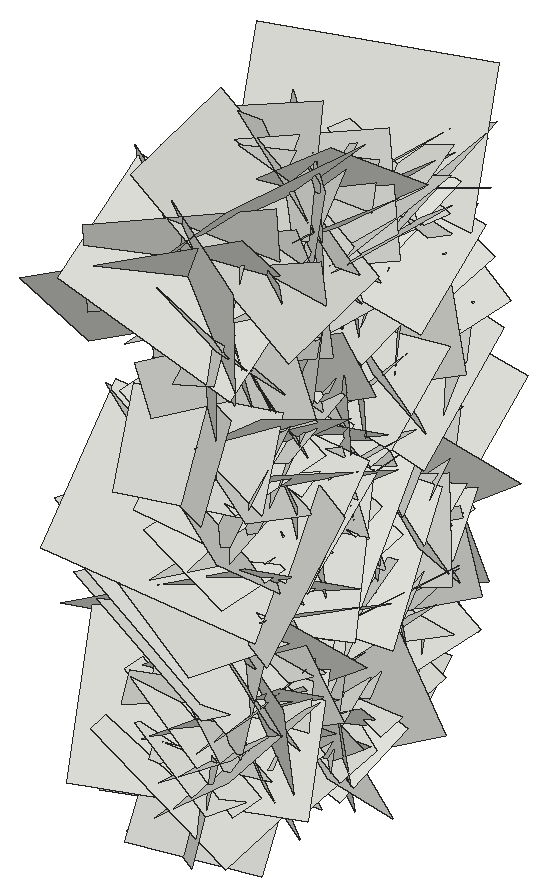
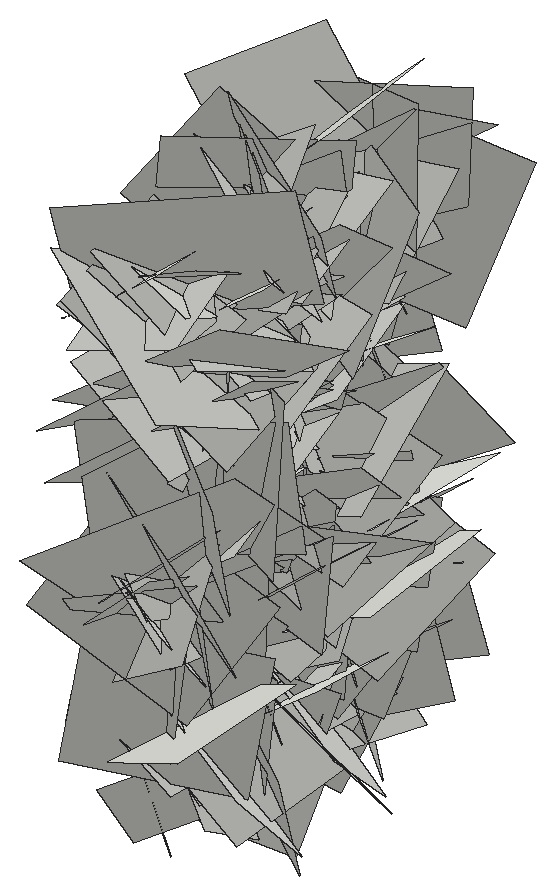
# SketchUp Ruby script. Lengths in inches.
U = 1.inch
M = Sketchup.active_model
def pt(a) = Geom::Point3d.new(a.map { |v| v * U })
def face(e, loops, mat)
  f = e.add_face(loops[0].map { |a| pt(a) })
  loops[1..].each { |l| e.add_face(l.map { |a| pt(a) }).erase! }
  f.material = f.back_material = mat if mat
  f
end
# faces: each face lists its corners as indices into pts; further lists are holes
def faces(e, pts, list, mat = nil) = list.each { |f| face(e, (f[0].is_a?(Array) ? f : [f]).map { |l| l.map { |i| pts[i] } }, mat) }
# xy, xz, yz: faces in a plane at the given z, y or x. An outline is a flat list of corners, or four numbers for a rectangle; further outlines are holes
def ring(l) = l.size == 4 ? [[l[0], l[1]], [l[2], l[1]], [l[2], l[3]], [l[0], l[3]]] : l.each_slice(2).to_a
def flat(e, list, mat, &to3) = list.each { |f| face(e, (f[0].is_a?(Array) ? f : [f]).map { |l| ring(l).map { |u, v| to3.(u, v) } }, mat) }
def xy(e, z, list, mat = nil) = flat(e, list, mat) { |x, y| [x, y, z] }
def xz(e, y, list, mat = nil) = flat(e, list, mat) { |x, z| [x, y, z] }
def yz(e, x, list, mat = nil) = flat(e, list, mat) { |y, z| [x, y, z] }
def lines(e, pts, list) = list.each { |a, b| e.add_line(pt(pts[a]), pt(pts[b])) }
# prism: a flat outline (further loops are holes) pulled along v
def prism(e, loops, v, mat = nil)
  f = face(e, loops, mat); d = Geom::Vector3d.new(v.map { |x| x * U })
  f.pushpull(f.normal.samedirection?(d) ? d.length : -d.length)
end
def box(e, o, s, mat = nil) = prism(e, [[o, [o[0] + s[0], o[1], o[2]], [o[0] + s[0], o[1] + s[1], o[2]], [o[0], o[1] + s[1], o[2]]]], [0, 0, s[2]], mat)
def at(x, y, z, deg = 0) = Geom::Transformation.translation(pt([x, y, z])) * Geom::Transformation.rotation(ORIGIN, Z_AXIS, deg.degrees)
def axes(o, x, y, z) = Geom::Transformation.new([*x, 0, *y, 0, *z, 0, *pt(o).to_a, 1])
def part(name) = M.definitions.add(name)
# library, detail: a bought-in or finely detailed component or shape, given as its bounding box
def library(name, o, s) = part(name).tap { |d| box(d.entities, o, s) }
def detail(e, o, s) = box(e.add_group.entities, o, s)
def put(e, d, t, mat = nil) = e.add_instance(d, t).tap { |i| i.material = mat if mat }
def group(e, t, mat = nil) = e.add_group.tap { |g| g.transformation = t; g.material = mat if mat }.entities
root = M.entities
c1 = part("Component\#6")
p = [[0.01,0,0],[0,3.24,4.54],[4.32,3.24,4.54],[4.33,0,0]]
faces(c1.entities,p,[[0,1,2,3]])
put(root,c1,axes([404.88,182.27,16.13],[-0.23771,-0.47409,1.27281],[-0.00404,1.29026,0.47991],[-1.43973,0.07465,-0.2115]))
put(root,c1,axes([404.88,189.11,8.53],[-0.25892,-1.11224,-0.53402],[-0.14932,-0.51568,1.13849],[-1.29927,0.28091,-0.02442]))
put(root,c1,axes([404.88,193.85,16.74],[-0.30124,-1.14539,-0.57535],[0.00001,-0.58933,1.17321],[-1.35869,0.25394,0.12757]))
put(root,c1,axes([404.88,184.58,6.82],[-0.16596,-1.29847,0.14138],[-0.0614,0.14916,1.30572],[-1.38315,0.14917,-0.07492]))
put(root,c1,axes([404.88,183.54,2.14],[-0.03864,0.84179,0.92004],[-0.33491,0.88417,-0.82148],[-1.27872,-0.257,0.18735]))
put(root,c1,axes([404.88,180.76,23.09],[-0.06995,0.91309,-0.96842],[-0.10566,-0.97028,-0.90805],[-1.4069,0.02747,0.11634]))
put(root,c1,axes([404.88,187.39,3.1875],[-0.10139,0.89849,0.89189],[-0.1671,0.87902,-0.90243],[-1.33152,-0.17873,0.04534]))
put(root,c1,axes([404.88,189.55,17.94],[-0.16397,-1.09761,-0.83604],[0.11999,-0.84854,1.09307],[-1.45761,0.05363,0.18403]))
put(root,c1,axes([404.88,193.03,3.2],[-0.23388,-1.096,0.27231],[-0.13541,0.2999,1.10354],[-1.1894,0.18138,-0.17918]))
put(root,c1,axes([404.88,184.34,4.6],[-0.11485,-1.15497,0.26483],[-0.19184,0.27894,1.14248],[-1.2413,0.06375,-0.20107]))
put(root,c1,axes([404.88,186.39,13.5625],[-0.22643,-0.80881,0.81079],[-0.0736,0.83241,0.81208],[-1.21171,0.10058,-0.20084]))
put(root,c1,axes([404.88,188.34,12.62],[-0.20954,0.481,1.15591],[0.07101,1.17261,-0.47649],[-1.32521,-0.01322,-0.2083]))
put(root,c1,axes([404.88,184,8.18],[0.02134,-1.06466,0.81449],[-0.04088,0.81378,1.06469],[-1.42032,-0.03942,-0.01841]))
put(root,c1,axes([404.88,184.23,21.55],[-0.30098,0.54789,0.85036],[-0.10123,0.86476,-0.58905],[-1.06749,-0.23649,-0.1839]))
put(root,c1,axes([404.88,183.88,15.08],[0.0404,1.11797,-0.62329],[-0.16276,-0.61507,-1.11262],[-1.34698,0.10785,0.11575]))
put(root,c1,axes([404.88,195.54,11.625],[-0.04246,-1.00606,-0.92627],[0.11693,-0.92602,1.00103],[-1.44486,-0.04538,0.10823]))
put(root,c1,axes([404.88,186.02,17.55],[-0.12484,-0.91824,0.67786],[-0.09261,0.68671,0.91505],[-1.20627,0.04231,-0.14041]))
put(root,c1,axes([404.88,185.87,11.99],[-0.00632,-0.88407,-1.06115],[0.10628,-1.05864,0.88141],[-1.46017,-0.07323,0.06874]))
put(root,c1,axes([404.88,192.77,15.58],[-0.03721,-0.16955,-1.17702],[-0.1418,-1.1695,0.17246],[-1.25252,0.13744,0.01545]))
put(root,c1,axes([404.88,186.66,10.07],[0.09303,-0.2424,1.37134],[0.00293,1.37409,0.24271],[-1.47615,-0.01254,0.08691]))
put(root,c1,axes([404.88,182.38,2.76],[-0.16715,0.82367,0.72398],[-0.09449,0.71938,-0.83785],[-1.15857,-0.1775,-0.03612]))
put(root,c1,axes([404.88,185.25,0.97],[-0.15144,0.45294,1.0525],[-0.02813,1.05906,-0.45936],[-1.21425,-0.08102,-0.12063]))
put(root,c1,axes([404.88,184.5,10.44],[-0.20009,0.552,-0.98447],[0.02572,-0.99592,-0.56307],[-1.1961,-0.11375,0.15258]))
put(root,c1,axes([404.88,180.93,10.86],[0.17521,1.15715,-0.62152],[-0.20897,-0.59747,-1.1648],[-1.37654,0.23798,0.09772]))
put(root,c1,axes([404.88,185.31,6.45],[0.03902,-0.20515,1.15818],[-0.22164,1.13915,0.20842],[-1.22693,-0.21231,-0.00082]))
put(root,c1,axes([404.88,183.02,16.38],[0.02893,-0.8566,0.75588],[-0.26219,0.73373,0.84043],[-1.18223,-0.18368,-0.16789]))
put(root,c1,axes([404.88,190.12,11.53],[0.21117,-0.99907,-0.90649],[-0.1512,-0.92678,0.99009],[-1.42194,-0.04983,-0.2399]))
put(root,c1,axes([404.88,188.7,21.97],[-0.14471,1.28216,-0.28655],[0.25359,-0.25902,-1.27293],[-1.36933,-0.18346,-0.20546]))
put(root,c1,axes([404.88,189.36,1.43],[0.09807,-1.35815,-0.14277],[0.05055,-0.1398,1.36078],[-1.44669,-0.09695,0.03787]))
put(root,c1,axes([404.88,194.04,23.84],[0.15699,-0.54259,-1.24113],[-0.03696,-1.24964,0.54215],[-1.43535,-0.02717,-0.14971]))
put(root,c1,axes([404.88,188.23,7.57],[-0.0913,-1.12353,0.75234],[0.27462,0.72618,1.11413],[-1.40673,0.21468,0.16867]))
put(root,c1,axes([404.88,192.17,8.01],[-0.17438,0.53527,-0.89237],[-0.02164,-0.90494,-0.53904],[-1.10282,-0.06688,0.15168]))
put(root,c1,axes([404.88,182.53,23.48],[-0.24403,0.37129,-0.99391],[0.1038,-1.00526,-0.39821],[-1.11985,-0.17408,0.17968]))
put(root,c1,axes([404.88,182.44,13.63],[0.1579,1.28482,-0.45217],[0.02165,-0.45692,-1.2916],[-1.44363,0.13368,-0.06883]))
put(root,c1,axes([404.88,189.08,9.2],[0.13088,0.55221,1.09741],[-0.12619,1.10312,-0.54169],[-1.29609,-0.05164,0.16356]))
put(root,c1,axes([404.88,187.9375,5.11],[-0.04973,-1.23753,-0.07043],[0.13139,-0.07481,1.23194],[-1.30732,0.03956,0.12649]))
put(root,c1,axes([400.91,190.35,18.26],[-0.16101,-0.65287,0.16772],[-0.08445,0.18811,0.66008],[0.7095,-0.12576,0.11663]))
put(root,c1,axes([404.88,186.43,6.6],[0.00451,1.27416,-0.10814],[0.14001,-0.108,-1.26731],[-1.34821,-0.00695,-0.13197]))
put(root,c1,axes([404.88,185.36,5.79],[-0.02078,-1.22604,-0.15411],[0.11589,-0.15525,1.22117],[-1.3047,0.00574,0.11093]))
put(root,c1,axes([404.88,188.68,19.83],[0.08458,1.11358,0.50301],[0.01593,0.50315,-1.11627],[-1.29513,0.07891,0.01912]))
put(root,c1,axes([404.88,186.13,19.34],[-0.13168,0.96657,0.23982],[-0.01085,0.24043,-0.97432],[-1.05558,-0.12304,-0.0199]))
put(root,c1,axes([400.91,191.11,1.26],[-0.04561,-0.57908,-0.31344],[-0.1156,-0.3035,0.57569],[0.68833,-0.08935,0.07592]))
put(root,c1,axes([404.88,187.26,9.21],[-0.06299,-0.71122,-0.64775],[-0.16214,-0.63375,0.70987],[-1.00673,0.14657,-0.0738]))
put(root,c1,axes([404.88,187.48,17.59],[0.04794,-0.78864,0.66349],[-0.19289,0.64758,0.78214],[-1.07529,-0.15133,-0.11072]))
put(root,c1,axes([404.88,180.4,17.125],[0.23878,-0.31981,1.17522],[-0.15258,1.17979,0.34864],[-1.28199,-0.19998,0.17739]))
put(root,c1,axes([404.88,185.11,13.22],[-0.08906,-0.95701,-0.12674],[-0.0585,-0.12225,0.95969],[-1.02162,0.09043,-0.0439]))
put(root,c1,axes([404.88,191.125,9.45],[0.23474,-0.88576,-0.93612],[-0.00151,-0.95001,0.89856],[-1.36608,-0.15116,-0.16185]))
put(root,c1,axes([404.88,184.05,20.67],[-0.10102,0.73684,0.6989],[0.04073,0.70408,-0.73707],[-1.07574,-0.04254,-0.09354]))
put(root,c1,axes([404.88,181.08,20.02],[0.00536,1.00575,0.03656],[-0.10796,0.03689,-1.00058],[-1.06133,0.00133,0.10197]))
put(root,c1,axes([404.88,185.52,6.2],[0.2751,-0.65276,-1.16933],[0.03559,-1.18754,0.67037],[-1.41909,-0.15632,-0.20987]))
put(root,c1,axes([400.91,188.8,6.44],[-0.14743,-0.18272,-0.74199],[-0.06403,-0.74919,0.19581],[0.80747,-0.09277,-0.11994]))
put(root,c1,axes([404.88,179.32,18.3],[-0.15069,0.54422,0.74866],[0.00735,0.75804,-0.54972],[-0.98107,-0.07791,-0.11911]))
put(root,c1,axes([404.88,184.31,4.6],[-0.1576,-0.1516,-1.0147],[0.15202,-1.0183,0.13112],[-1.07684,-0.12157,0.16702]))
put(root,c1,axes([400.91,186.3,8.38],[0.07617,0.47932,0.41871],[-0.13681,0.42359,-0.46276],[0.66062,0.03245,-0.14411]))
put(root,c1,axes([404.88,184.41,20.14],[0.03821,-1.03167,-0.60174],[0.15497,-0.59368,1.0266],[-1.25647,-0.1046,0.10832]))
put(root,c1,axes([404.88,194.3,13.93],[0.22437,-1.23478,-0.60854],[0.19245,-0.58527,1.25072],[-1.44644,-0.26941,0.07201]))
put(root,c1,axes([400.91,187.98,11.49],[-0.12716,0.81746,0.20835],[-0.15,0.18797,-0.81896],[0.88154,0.1499,-0.10929]))
put(root,c1,axes([400.91,186.0625,6.1],[-0.08854,0.52684,0.45627],[0.00383,0.45985,-0.53032],[0.73876,0.06076,0.05744]))
put(root,c1,axes([404.88,181.29,16.68],[-0.08133,-0.245,0.96212],[0.05676,0.96256,0.24939],[-1.05086,0.07095,-0.06099]))
put(root,c1,axes([404.88,184.19,13.53],[-0.08078,-0.49886,0.79857],[-0.01528,0.8017,0.49945],[-0.99796,0.02811,-0.07229]))
put(root,c1,axes([404.88,187.61,11.62],[0.28203,-0.58282,-1.12773],[-0.01249,-1.15332,0.59327],[-1.34554,-0.11146,-0.24188]))
put(root,c1,axes([400.91,183.1,18.89],[-0.1435,0.17311,-0.85276],[-0.14536,-0.85648,-0.1521],[0.91084,-0.10941,-0.15862]))
put(root,c1,axes([400.91,183.83,7.3125],[-0.02805,0.62389,-0.09529],[0.05665,-0.09282,-0.62253],[0.66659,0.03414,0.0489]))
put(root,c1,axes([404.88,184.51,1.15],[0.01173,-1.06899,-0.22188],[0.10644,-0.21996,1.06472],[-1.15237,-0.0312,0.09608]))
put(root,c1,axes([404.88,186.9375,3.03],[-0.11563,0.62873,-0.58509],[-0.05581,-0.59358,-0.62803],[-0.90867,-0.04354,0.11303]))
put(root,c1,axes([400.91,189.45,1.42],[0.1039,0.30381,0.53974],[-0.07033,0.54846,-0.29667],[0.65275,0.01074,-0.11787]))
put(root,c1,axes([400.91,184.54,3.47],[-0.05739,0.5962,-0.42459],[-0.0201,-0.42675,-0.59681],[0.77559,0.03305,-0.04688]))
put(root,c1,axes([404.88,185.64,19.96],[0.2349,1.07139,0.39402],[-0.08081,0.41437,-1.08385],[-1.20734,0.18072,0.1492]))
put(root,c1,axes([404.88,186.72,4.72],[0.08241,-0.91883,0.29273],[-0.13826,0.28096,0.91654],[-1.0128,-0.11312,-0.1013]))
put(root,c1,axes([404.88,190.33,17.67],[-0.17424,0.82504,0.17436],[0.04616,0.18571,-0.83769],[-0.89267,-0.15144,-0.07735]))
put(root,c1,axes([404.88,179.97,24.47],[0.23304,1.36821,0.06434],[0.25904,0.02493,-1.36533],[-1.42861,0.2277,-0.23708]))
put(root,c1,axes([400.91,184.43,15.42],[-0.12844,-0.04329,0.74472],[0.08874,0.74892,0.05716],[0.78574,-0.09166,0.11528]))
put(root,c1,axes([404.88,189.57,16.9],[-0.06471,0.53395,-0.71324],[-0.01751,-0.71546,-0.53421],[-0.94426,-0.02333,0.05878]))
put(root,c1,axes([404.88,191,16.96],[0.17643,-1.14926,-0.11809],[0.05518,-0.11173,1.16072],[-1.22339,-0.17078,0.03532]))
put(root,c1,axes([400.91,186.92,8.78],[-0.10246,-0.30095,0.75916],[-0.04625,0.76527,0.29782],[0.86439,0.00528,0.10592]))
put(root,c1,axes([404.88,180.14,11.99],[0.0212,0.75168,0.8023],[0.17372,0.79143,-0.74558],[-1.15236,0.13314,-0.09764]))
put(root,c1,axes([404.88,185.08,2.16],[-0.06404,-1.02262,-0.11109],[0.17979,-0.11966,1.00929],[-1.07543,0.04089,0.17535]))
put(root,c1,axes([404.88,187.17,12.95],[0.05814,-0.16279,1.09674],[0.14666,1.09051,0.15494],[-1.1661,0.12904,0.07417]))
put(root,c1,axes([404.88,187.85,22.99],[-0.09057,-0.06637,-0.91857],[0.07612,-0.92019,0.05981],[-0.97325,-0.06579,0.09016]))
put(root,c1,axes([400.91,183.375,2.21],[0.01982,-0.33114,-0.74136],[-0.16849,-0.7287,0.32148],[0.84401,-0.13769,0.08159]))
put(root,c1,axes([400.91,192.83,7.86],[0.1126,-0.65912,-0.17655],[-0.1088,-0.19208,0.65534],[0.71507,0.07456,0.12751]))
put(root,c1,axes([404.88,183.46,7.83],[0.1867,0.36795,-0.96583],[-0.13041,-0.96532,-0.39019],[-1.08777,0.17888,-0.11899]))
put(root,c1,axes([404.88,186.63,-0.64],[0.14781,-0.37723,1.01914],[0.01271,1.02797,0.37886],[-1.15185,-0.03706,0.13496]))
put(root,c1,axes([404.88,183.61,1.59],[-0.06331,-0.78644,0.46242],[0.03597,0.46118,0.7887],[-0.96639,0.06869,-0.00094]))
put(root,c1,axes([404.88,185.25,15.47],[-0.04372,0.77316,0.71524],[0.20224,0.70943,-0.75587],[-1.09798,0.09988,-0.16771]))
put(root,c1,axes([404.88,185.13,2.21],[-0.09174,0.69928,0.36],[-0.10121,0.35015,-0.7031],[-0.82753,-0.12035,0.04608]))
put(root,c1,axes([400.91,192.38,19.24],[0.04943,-0.7355,0.057],[-0.07325,0.05251,0.73407],[0.77853,0.05163,0.06545]))
put(root,c1,axes([404.88,181.6,11.88],[-0.05183,0.72565,0.67247],[0.15864,0.67097,-0.71314],[-1.03662,0.0664,-0.14276]))
put(root,c1,axes([400.91,185.26,12.26],[-0.159,0.84642,0.10737],[0.04855,0.11685,-0.85715],[0.9031,0.14274,0.06498]))
put(root,c1,axes([400.91,185.94,13.1875],[-0.12339,0.16979,-0.82402],[0.01755,-0.83125,-0.17361],[0.89164,0.03986,-0.11061]))
put(root,c1,axes([400.91,183.19,13.8],[-0.02762,0.65605,0.3231],[0.06014,0.32414,-0.6536],[0.77284,-0.00178,0.06241]))
put(root,c1,axes([404.88,184.53,11.29],[0.10396,-0.95246,0.37472],[0.04499,0.37989,0.95451],[-1.084,-0.07558,0.07555]))
put(root,c1,axes([404.88,192.08,20.31],[-0.05296,-0.67773,-0.30339],[-0.1724,-0.2867,0.66724],[-0.76797,0.11109,-0.12886]))
put(root,c1,axes([400.91,192.03,8.33],[-0.03388,0.22508,-0.86549],[-0.13142,-0.8588,-0.21876],[0.93879,-0.1121,-0.06186]))
put(root,c1,axes([400.91,185.14,8.49],[0.08576,-0.66072,-0.04627],[0.0456,-0.04128,0.66459],[0.70059,0.08356,-0.03759]))
put(root,c1,axes([400.91,183.28,17.73],[-0.09647,-0.26045,0.74001],[0.11879,0.73302,0.27177],[0.82305,-0.13632,0.04751]))
put(root,c1,axes([400.91,193.37,9.31],[-0.05697,-0.46717,-0.61186],[0.09106,-0.61316,0.46062],[0.81091,0.03603,-0.09471]))
put(root,c1,axes([400.91,191.46,9.82],[-0.08538,-0.06629,-0.92063],[-0.09555,-0.91915,0.07407],[0.97372,-0.09601,-0.07345]))
put(root,c1,axes([400.91,191.35,2.27],[-0.06694,-0.86655,-0.10749],[-0.04783,-0.10439,0.86806],[0.92435,-0.06816,0.03713]))
put(root,c1,axes([400.91,190.84,12.42],[0.00848,-0.77925,-0.15089],[-0.03038,-0.15108,0.77873],[0.8408,0.0024,0.02966]))
put(root,c1,axes([400.91,182.98,9.92],[0.09782,-0.62966,-0.10425],[0.08997,-0.09229,0.63256],[0.67052,0.10424,-0.06967]))
put(root,c1,axes([400.91,180.19,4.07],[0.08532,0.68038,-0.07405],[0.04058,-0.07892,-0.68351],[0.72433,-0.07573,0.04702]))
put(root,c1,axes([400.91,183.91,5.17],[-0.1157,0.58195,-0.7538],[-0.08085,-0.76164,-0.57696],[1.0062,0.00571,-0.13304]))
put(root,c1,axes([400.91,182.875,15.8],[-0.04284,-0.30855,-0.78276],[-0.017,-0.78324,0.30957],[0.8917,-0.02976,-0.0317]))
put(root,c1,axes([404.88,184.33,2.33],[0.23495,-0.78095,0.69461],[-0.033,0.70481,0.80235],[-1.10738,-0.18669,0.12346]))
put(root,c1,axes([404.88,189.86,21.06],[0.09411,0.75469,-0.30292],[-0.23058,-0.27158,-0.74036],[-0.83059,0.16091,0.17121]))
put(root,c1,axes([404.88,189.65,5.54],[-0.06955,0.77959,0.08211],[-0.00823,0.08175,-0.78235],[-0.8309,-0.06607,0.00087]))
put(root,c1,axes([404.88,192.04,5.47],[0.24252,-0.79203,0.72828],[0.0092,0.7459,0.80846],[-1.14049,-0.1624,0.16139]))
put(root,c1,axes([404.88,184.16,21.8125],[0.07155,0.99261,-0.10082],[0.11355,-0.10768,-0.9884],[-1.05147,0.05592,-0.1136]))
put(root,c1,axes([400.91,184.68,7.1],[-0.07537,-0.21143,-0.85755],[-0.01444,-0.85996,0.21315],[0.93612,-0.03029,-0.06575]))
put(root,c1,axes([400.91,187.95,18.35],[-0.24952,-0.85217,0.60628],[-0.01294,0.62364,0.87183],[1.1085,-0.18454,0.14665]))
put(root,c1,axes([404.88,188.38,23.95],[0.14683,-0.05211,-1.06804],[0.1506,-1.06652,0.07046],[-1.12342,-0.14978,-0.13015]))
put(root,c1,axes([400.91,188.38,23.95],[-0.14683,-0.05211,-1.06804],[-0.1506,-1.06652,0.07046],[1.12342,-0.14978,-0.13015]))
put(root,c1,axes([404.88,187.95,18.35],[0.24952,-0.85217,0.60628],[0.01294,0.62364,0.87183],[-1.1085,-0.18454,0.14665]))
put(root,c1,axes([404.88,184.68,7.1],[0.07537,-0.21143,-0.85755],[0.01444,-0.85996,0.21315],[-0.93612,-0.03029,-0.06575]))
put(root,c1,axes([400.91,184.16,21.8125],[-0.07155,0.99261,-0.10082],[-0.11355,-0.10768,-0.9884],[1.05147,0.05592,-0.1136]))
put(root,c1,axes([400.91,192.04,5.47],[-0.24252,-0.79203,0.72828],[-0.0092,0.7459,0.80846],[1.14049,-0.1624,0.16139]))
put(root,c1,axes([400.91,189.65,5.54],[0.06955,0.77959,0.08211],[0.00823,0.08175,-0.78235],[0.8309,-0.06607,0.00087]))
put(root,c1,axes([400.91,189.86,21.06],[-0.09411,0.75469,-0.30292],[0.23058,-0.27158,-0.74036],[0.83059,0.16091,0.17121]))
put(root,c1,axes([400.91,184.33,2.33],[-0.23495,-0.78095,0.69461],[0.033,0.70481,0.80235],[1.10738,-0.18669,0.12346]))
put(root,c1,axes([404.88,182.875,15.8],[0.04284,-0.30855,-0.78276],[0.017,-0.78324,0.30957],[-0.8917,-0.02976,-0.0317]))
put(root,c1,axes([404.88,183.91,5.17],[0.1157,0.58195,-0.7538],[0.08085,-0.76164,-0.57696],[-1.0062,0.00571,-0.13304]))
put(root,c1,axes([404.88,180.19,4.07],[-0.08532,0.68038,-0.07405],[-0.04058,-0.07892,-0.68351],[-0.72433,-0.07573,0.04702]))
put(root,c1,axes([404.88,182.98,9.92],[-0.09782,-0.62966,-0.10425],[-0.08997,-0.09229,0.63256],[-0.67052,0.10424,-0.06967]))
put(root,c1,axes([404.88,190.84,12.42],[-0.00848,-0.77925,-0.15089],[0.03038,-0.15108,0.77873],[-0.8408,0.0024,0.02966]))
put(root,c1,axes([404.88,191.35,2.27],[0.06694,-0.86655,-0.10749],[0.04783,-0.10439,0.86806],[-0.92435,-0.06816,0.03713]))
put(root,c1,axes([404.88,191.46,9.82],[0.08538,-0.06629,-0.92063],[0.09555,-0.91915,0.07407],[-0.97372,-0.09601,-0.07345]))
put(root,c1,axes([404.88,193.37,9.31],[0.05697,-0.46717,-0.61186],[-0.09106,-0.61316,0.46062],[-0.81091,0.03603,-0.09471]))
put(root,c1,axes([404.88,183.28,17.73],[0.09647,-0.26045,0.74001],[-0.11879,0.73302,0.27177],[-0.82305,-0.13632,0.04751]))
put(root,c1,axes([404.88,185.14,8.49],[-0.08576,-0.66072,-0.04627],[-0.0456,-0.04128,0.66459],[-0.70059,0.08356,-0.03759]))
put(root,c1,axes([404.88,192.03,8.33],[0.03388,0.22508,-0.86549],[0.13142,-0.8588,-0.21876],[-0.93879,-0.1121,-0.06186]))
put(root,c1,axes([400.91,192.08,20.31],[0.05296,-0.67773,-0.30339],[0.1724,-0.2867,0.66724],[0.76797,0.11109,-0.12886]))
put(root,c1,axes([400.91,184.53,11.29],[-0.10396,-0.95246,0.37472],[-0.04499,0.37989,0.95451],[1.084,-0.07558,0.07555]))
put(root,c1,axes([404.88,183.19,13.8],[0.02762,0.65605,0.3231],[-0.06014,0.32414,-0.6536],[-0.77284,-0.00178,0.06241]))
put(root,c1,axes([404.88,185.94,13.1875],[0.12339,0.16979,-0.82402],[-0.01755,-0.83125,-0.17361],[-0.89164,0.03986,-0.11061]))
put(root,c1,axes([404.88,185.26,12.26],[0.159,0.84642,0.10737],[-0.04855,0.11685,-0.85715],[-0.9031,0.14274,0.06498]))
put(root,c1,axes([400.91,181.6,11.88],[0.05183,0.72565,0.67247],[-0.15864,0.67097,-0.71314],[1.03662,0.0664,-0.14276]))
put(root,c1,axes([404.88,192.38,19.24],[-0.04943,-0.7355,0.057],[0.07325,0.05251,0.73407],[-0.77853,0.05163,0.06545]))
put(root,c1,axes([400.91,185.13,2.21],[0.09174,0.69928,0.36],[0.10121,0.35015,-0.7031],[0.82753,-0.12035,0.04608]))
put(root,c1,axes([400.91,185.25,15.47],[0.04372,0.77316,0.71524],[-0.20224,0.70943,-0.75587],[1.09798,0.09988,-0.16771]))
put(root,c1,axes([400.91,183.61,1.59],[0.06331,-0.78644,0.46242],[-0.03597,0.46118,0.7887],[0.96639,0.06869,-0.00094]))
put(root,c1,axes([400.91,186.63,-0.64],[-0.14781,-0.37723,1.01914],[-0.01271,1.02797,0.37886],[1.15185,-0.03706,0.13496]))
put(root,c1,axes([400.91,183.46,7.83],[-0.1867,0.36795,-0.96583],[0.13041,-0.96532,-0.39019],[1.08777,0.17888,-0.11899]))
put(root,c1,axes([404.88,192.83,7.86],[-0.1126,-0.65912,-0.17655],[0.1088,-0.19208,0.65534],[-0.71507,0.07456,0.12751]))
put(root,c1,axes([404.88,183.375,2.21],[-0.01982,-0.33114,-0.74136],[0.16849,-0.7287,0.32148],[-0.84401,-0.13769,0.08159]))
put(root,c1,axes([400.91,187.85,22.99],[0.09057,-0.06637,-0.91857],[-0.07612,-0.92019,0.05981],[0.97325,-0.06579,0.09016]))
put(root,c1,axes([400.91,187.17,12.95],[-0.05814,-0.16279,1.09674],[-0.14666,1.09051,0.15494],[1.1661,0.12904,0.07417]))
put(root,c1,axes([400.91,185.08,2.16],[0.06404,-1.02262,-0.11109],[-0.17979,-0.11966,1.00929],[1.07543,0.04089,0.17535]))
put(root,c1,axes([400.91,180.14,11.99],[-0.0212,0.75168,0.8023],[-0.17372,0.79143,-0.74558],[1.15236,0.13314,-0.09764]))
put(root,c1,axes([404.88,186.92,8.78],[0.10246,-0.30095,0.75916],[0.04625,0.76527,0.29782],[-0.86439,0.00528,0.10592]))
put(root,c1,axes([400.91,191,16.96],[-0.17643,-1.14926,-0.11809],[-0.05518,-0.11173,1.16072],[1.22339,-0.17078,0.03532]))
put(root,c1,axes([400.91,189.57,16.9],[0.06471,0.53395,-0.71324],[0.01751,-0.71546,-0.53421],[0.94426,-0.02333,0.05878]))
put(root,c1,axes([404.88,184.43,15.42],[0.12844,-0.04329,0.74472],[-0.08874,0.74892,0.05716],[-0.78574,-0.09166,0.11528]))
put(root,c1,axes([400.91,179.97,24.47],[-0.23304,1.36821,0.06434],[-0.25904,0.02493,-1.36533],[1.42861,0.2277,-0.23708]))
put(root,c1,axes([400.91,190.33,17.67],[0.17424,0.82504,0.17436],[-0.04616,0.18571,-0.83769],[0.89267,-0.15144,-0.07735]))
put(root,c1,axes([400.91,186.72,4.72],[-0.08241,-0.91883,0.29273],[0.13826,0.28096,0.91654],[1.0128,-0.11312,-0.1013]))
put(root,c1,axes([400.91,185.64,19.96],[-0.2349,1.07139,0.39402],[0.08081,0.41437,-1.08385],[1.20734,0.18072,0.1492]))
put(root,c1,axes([404.88,184.54,3.47],[0.05739,0.5962,-0.42459],[0.0201,-0.42675,-0.59681],[-0.77559,0.03305,-0.04688]))
put(root,c1,axes([404.88,189.45,1.42],[-0.1039,0.30381,0.53974],[0.07033,0.54846,-0.29667],[-0.65275,0.01074,-0.11787]))
put(root,c1,axes([400.91,186.9375,3.03],[0.11563,0.62873,-0.58509],[0.05581,-0.59358,-0.62803],[0.90867,-0.04354,0.11303]))
put(root,c1,axes([400.91,184.51,1.15],[-0.01173,-1.06899,-0.22188],[-0.10644,-0.21996,1.06472],[1.15237,-0.0312,0.09608]))
put(root,c1,axes([404.88,183.83,7.3125],[0.02805,0.62389,-0.09529],[-0.05665,-0.09282,-0.62253],[-0.66659,0.03414,0.0489]))
put(root,c1,axes([404.88,183.1,18.89],[0.1435,0.17311,-0.85276],[0.14536,-0.85648,-0.1521],[-0.91084,-0.10941,-0.15862]))
put(root,c1,axes([400.91,187.61,11.62],[-0.28203,-0.58282,-1.12773],[0.01249,-1.15332,0.59327],[1.34554,-0.11146,-0.24188]))
put(root,c1,axes([400.91,184.19,13.53],[0.08078,-0.49886,0.79857],[0.01528,0.8017,0.49945],[0.99796,0.02811,-0.07229]))
put(root,c1,axes([400.91,181.29,16.68],[0.08133,-0.245,0.96212],[-0.05676,0.96256,0.24939],[1.05086,0.07095,-0.06099]))
put(root,c1,axes([404.88,186.0625,6.1],[0.08854,0.52684,0.45627],[-0.00383,0.45985,-0.53032],[-0.73876,0.06076,0.05744]))
put(root,c1,axes([404.88,187.98,11.49],[0.12716,0.81746,0.20835],[0.15,0.18797,-0.81896],[-0.88154,0.1499,-0.10929]))
